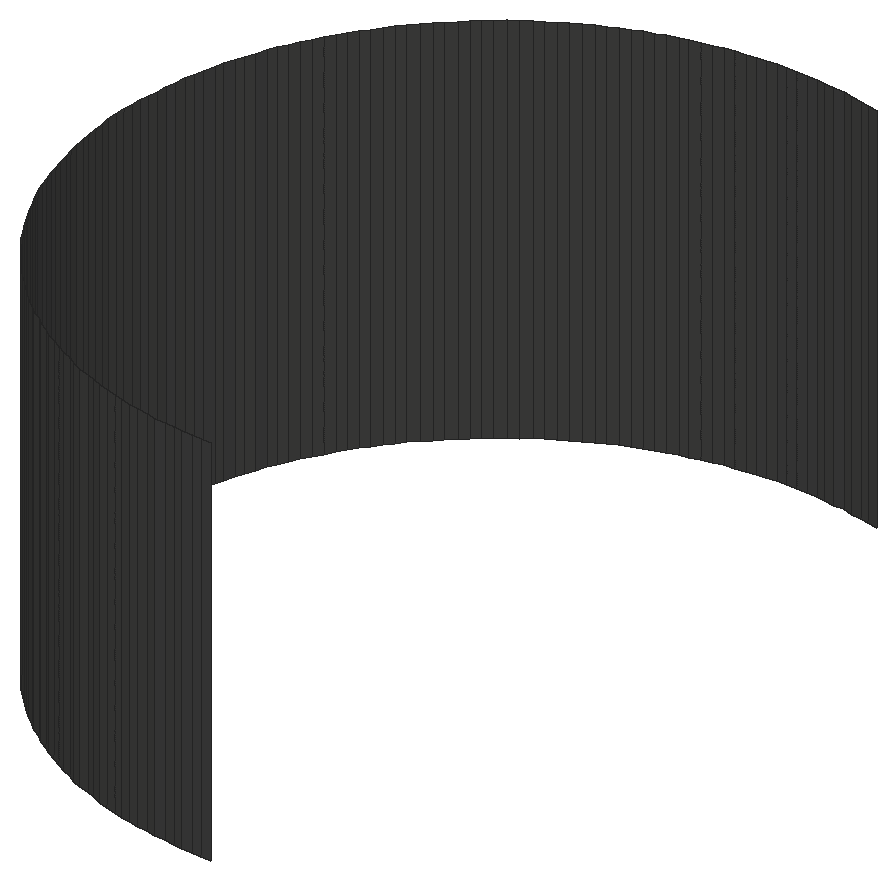
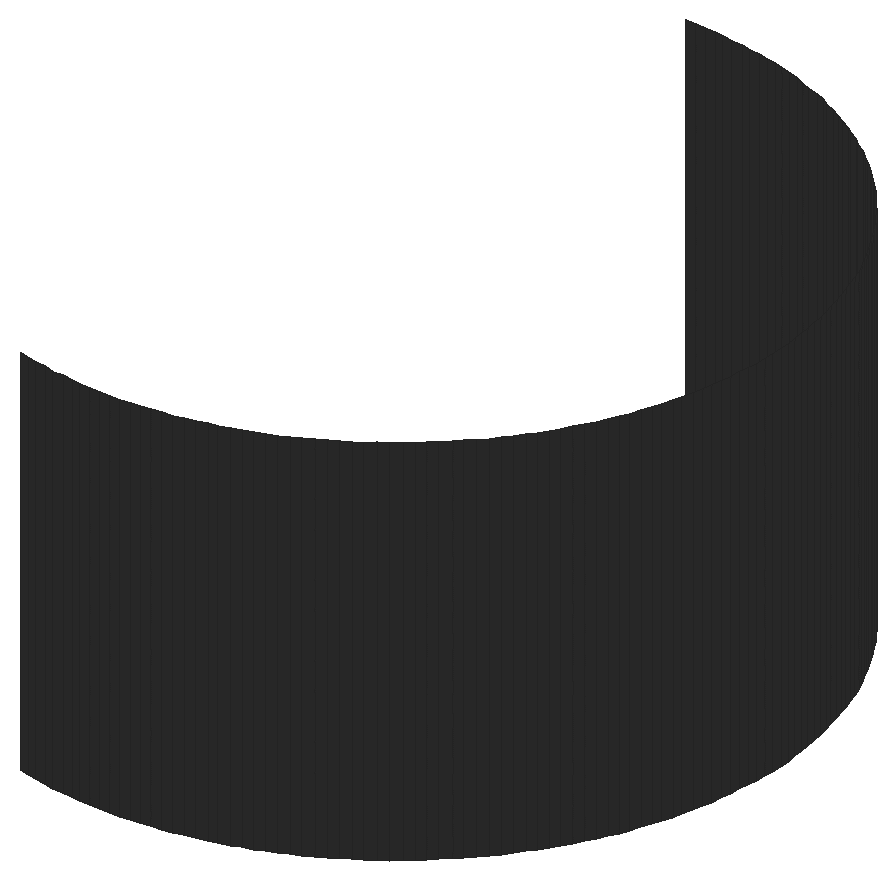
# SketchUp Ruby script. Lengths in inches.
U = 1.inch
M = Sketchup.active_model
def pt(a) = Geom::Point3d.new(a.map { |v| v * U })
def face(e, loops, mat)
  f = e.add_face(loops[0].map { |a| pt(a) })
  loops[1..].each { |l| e.add_face(l.map { |a| pt(a) }).erase! }
  f.material = f.back_material = mat if mat
  f
end
# faces: each face lists its corners as indices into pts; further lists are holes
def faces(e, pts, list, mat = nil) = list.each { |f| face(e, (f[0].is_a?(Array) ? f : [f]).map { |l| l.map { |i| pts[i] } }, mat) }
# xy, xz, yz: faces in a plane at the given z, y or x. An outline is a flat list of corners, or four numbers for a rectangle; further outlines are holes
def ring(l) = l.size == 4 ? [[l[0], l[1]], [l[2], l[1]], [l[2], l[3]], [l[0], l[3]]] : l.each_slice(2).to_a
def flat(e, list, mat, &to3) = list.each { |f| face(e, (f[0].is_a?(Array) ? f : [f]).map { |l| ring(l).map { |u, v| to3.(u, v) } }, mat) }
def xy(e, z, list, mat = nil) = flat(e, list, mat) { |x, y| [x, y, z] }
def xz(e, y, list, mat = nil) = flat(e, list, mat) { |x, z| [x, y, z] }
def yz(e, x, list, mat = nil) = flat(e, list, mat) { |y, z| [x, y, z] }
def lines(e, pts, list) = list.each { |a, b| e.add_line(pt(pts[a]), pt(pts[b])) }
# prism: a flat outline (further loops are holes) pulled along v
def prism(e, loops, v, mat = nil)
  f = face(e, loops, mat); d = Geom::Vector3d.new(v.map { |x| x * U })
  f.pushpull(f.normal.samedirection?(d) ? d.length : -d.length)
end
def box(e, o, s, mat = nil) = prism(e, [[o, [o[0] + s[0], o[1], o[2]], [o[0] + s[0], o[1] + s[1], o[2]], [o[0], o[1] + s[1], o[2]]]], [0, 0, s[2]], mat)
def at(x, y, z, deg = 0) = Geom::Transformation.translation(pt([x, y, z])) * Geom::Transformation.rotation(ORIGIN, Z_AXIS, deg.degrees)
def axes(o, x, y, z) = Geom::Transformation.new([*x, 0, *y, 0, *z, 0, *pt(o).to_a, 1])
def part(name) = M.definitions.add(name)
# library, detail: a bought-in or finely detailed component or shape, given as its bounding box
def library(name, o, s) = part(name).tap { |d| box(d.entities, o, s) }
def detail(e, o, s) = box(e.add_group.entities, o, s)
def put(e, d, t, mat = nil) = e.add_instance(d, t).tap { |i| i.material = mat if mat }
def group(e, t, mat = nil) = e.add_group.tap { |g| g.transformation = t; g.material = mat if mat }.entities
root = M.entities
M.materials.add("1448 AP 8253 RAVEN SONG").color = [64, 64, 63]
xz(root,217.5,[[117.99,471,118.07,474],[118.07,471,118.15,474],[118.15,471,118.23,474]],"1448 AP 8253 RAVEN SONG")
xz(root,217.52,[[117.76,471,117.84,474]],"1448 AP 8253 RAVEN SONG")
xz(root,223.48,[[118.44,471,118.52,474]],"1448 AP 8253 RAVEN SONG")
xz(root,223.5,[[117.97,471,118.05,474],[118.05,471,118.13,474],[118.13,471,118.21,474],[118.21,471,118.29,474]],"1448 AP 8253 RAVEN SONG")
yz(root,115.14,[[220.33,471,220.41,474],[220.41,471,220.49,474],[220.49,471,220.57,474],[220.57,471,220.65,474]],"1448 AP 8253 RAVEN SONG")
yz(root,115.16,[[220.8,471,220.88,474]],"1448 AP 8253 RAVEN SONG")
p = [[117.6,217.55,471],[117.53,217.5625,471],[117.53,217.5625,474],[117.6,217.55,474],[117.68,217.54,471],[117.68,217.54,474],
  [117.76,217.52,471],[117.76,217.52,474],[117.92,217.51,471],[117.84,217.52,471],[117.84,217.52,474],[117.92,217.51,474],
  [117.99,217.5,471],[117.99,217.5,474],[117.22,217.64,471],[117.15,217.67,471],[117.15,217.67,474],[117.22,217.64,474],
  [117.3,217.62,471],[117.3,217.62,474],[117.375,217.6,471],[117.375,217.6,474],[117.45,217.58,471],[117.45,217.58,474],
  [117,217.72,471],[116.93,217.75,471],[116.93,217.75,474],[117,217.72,474],[117.08,217.7,471],[117.08,217.7,474],
  [116.79,217.82,471],[116.72,217.86,471],[116.72,217.86,474],[116.79,217.82,474],[116.86,217.79,471],[116.86,217.79,474],
  [116.58,217.9375,471],[116.52,217.98,471],[116.52,217.98,474],[116.58,217.9375,474],[116.65,217.9,471],[116.65,217.9,474],
  [116.45,218.02,471],[116.39,218.07,471],[116.39,218.07,474],[116.45,218.02,474],[116.32,218.11,471],[116.32,218.11,474],
  [116.26,218.16,471],[116.26,218.16,474],[116.2,218.21,471],[116.14,218.26,471],[116.14,218.26,474],[116.2,218.21,474],
  [116.08,218.32,471],[116.03,218.37,471],[116.03,218.37,474],[116.08,218.32,474],[115.97,218.43,471],[115.92,218.48,471],
  [115.92,218.48,474],[115.97,218.43,474],[115.87,218.54,471],[115.82,218.6,471],[115.82,218.6,474],[115.87,218.54,474],
  [115.77,218.66,471],[115.77,218.66,474],[115.72,218.73,471],[115.72,218.73,474],[115.67,218.79,471],[115.67,218.79,474],
  [115.63,218.86,471],[115.63,218.86,474],[115.59,218.92,471],[115.55,218.99,471],[115.55,218.99,474],[115.59,218.92,474],
  [115.51,219.06,471],[115.51,219.06,474],[115.47,219.13,471],[115.4375,219.2,471],[115.4375,219.2,474],[115.47,219.13,474],
  [115.4,219.27,471],[115.4,219.27,474],[115.37,219.34,471],[115.34,219.41,471],[115.34,219.41,474],[115.37,219.34,474],
  [115.32,219.49,471],[115.32,219.49,474],[115.29,219.5625,471],[115.29,219.5625,474],[115.27,219.64,471],[115.25,219.71,471],
  [115.25,219.71,474],[115.27,219.64,474],[115.23,219.79,471],[115.23,219.79,474],[115.21,219.87,471],[115.21,219.87,474],
  [115.19,219.94,471],[115.19,219.94,474],[115.18,220.02,471],[115.18,220.02,474],[115.17,220.1,471],[115.17,220.1,474],
  [115.16,220.18,471],[115.16,220.18,474],[115.15,220.25,471],[115.15,220.25,474],[115.14,220.33,471],[115.14,220.33,474],
  [115.14,220.65,471],[115.15,220.72,471],[115.15,220.72,474],[115.14,220.65,474],[115.16,220.8,471],[115.16,220.8,474],
  [115.16,220.88,471],[115.18,220.96,471],[115.18,220.96,474],[115.16,220.88,474],[115.1875,221.04,471],[115.1875,221.04,474],
  [115.2,221.11,471],[115.2,221.11,474],[115.22,221.1875,471],[115.22,221.1875,474],[115.24,221.27,471],[115.24,221.27,474],
  [115.26,221.34,471],[115.26,221.34,474],[115.28,221.42,471],[115.28,221.42,474],[115.31,221.49,471],[115.31,221.49,474],
  [115.34,221.5625,471],[115.34,221.5625,474],[115.36,221.64,471],[115.36,221.64,474],[115.39,221.71,471],[115.39,221.71,474],
  [115.43,221.78,471],[115.43,221.78,474],[115.46,221.85,471],[115.46,221.85,474],[115.5,221.92,471],[115.5,221.92,474],
  [115.54,221.99,471],[115.54,221.99,474],[115.58,222.06,471],[115.58,222.06,474],[115.62,222.125,471],[115.62,222.125,474],
  [115.66,222.19,471],[115.66,222.19,474],[115.71,222.25,471],[115.71,222.25,474],[115.75,222.32,471],[115.75,222.32,474],
  [115.8,222.38,471],[115.8,222.38,474],[115.85,222.44,471],[115.85,222.44,474],[115.9,222.5,471],[115.9,222.5,474],
  [115.96,222.56,471],[115.96,222.56,474],[116.01,222.61,471],[116.01,222.61,474],[116.07,222.67,471],[116.07,222.67,474],
  [116.125,222.72,471],[116.125,222.72,474],[116.18,222.77,471],[116.18,222.77,474],[116.24,222.82,471],[116.24,222.82,474],
  [116.3,222.875,471],[116.3,222.875,474],[116.37,222.92,471],[116.37,222.92,474],[116.43,222.97,471],[116.43,222.97,474],
  [116.5,223.01,471],[116.5,223.01,474],[116.5625,223.05,471],[116.5625,223.05,474],[116.63,223.09,471],[116.63,223.09,474],
  [116.7,223.13,471],[116.7,223.13,474],[116.77,223.17,471],[116.77,223.17,474],[116.84,223.2,471],[116.84,223.2,474],
  [116.91,223.24,471],[116.91,223.24,474],[116.98,223.27,471],[116.98,223.27,474],[117.05,223.3,471],[117.05,223.3,474],
  [117.13,223.32,471],[117.13,223.32,474],[117.2,223.35,471],[117.2,223.35,474],[117.28,223.375,471],[117.28,223.375,474],
  [117.35,223.39,471],[117.35,223.39,474],[117.43,223.41,471],[117.43,223.41,474],[117.51,223.43,471],[117.51,223.43,474],
  [117.58,223.45,471],[117.58,223.45,474],[117.66,223.46,471],[117.66,223.46,474],[118.68,223.45,471],[118.75,223.4375,471],
  [118.75,223.4375,474],[118.68,223.45,474],[118.83,223.42,471],[118.83,223.42,474],[117.74,223.47,471],[117.74,223.47,474],
  [117.82,223.48,471],[117.82,223.48,474],[117.89,223.49,471],[117.89,223.49,474],[117.97,223.5,471],[117.97,223.5,474],
  [118.29,223.5,471],[118.36,223.49,471],[118.36,223.49,474],[118.29,223.5,474],[118.44,223.48,471],[118.44,223.48,474],
  [118.52,223.48,471],[118.6,223.46,471],[118.6,223.46,474],[118.52,223.48,474]]
faces(root,p,[[0,1,2,3],[4,0,3,5],[6,4,5,7],[8,9,10,11],[12,8,11,13],[14,15,16,17],[18,14,17,19],[20,18,19,21],
  [22,20,21,23],[1,22,23,2],[24,25,26,27],[28,24,27,29],[15,28,29,16],[30,31,32,33],[34,30,33,35],[25,34,35,26],
  [36,37,38,39],[31,40,41,32],[40,36,39,41],[42,43,44,45],[37,42,45,38],[43,46,47,44],[46,48,49,47],[50,51,52,53],
  [48,50,53,49],[54,55,56,57],[51,54,57,52],[58,59,60,61],[55,58,61,56],[62,63,64,65],[59,62,65,60],[63,66,67,64],
  [66,68,69,67],[68,70,71,69],[70,72,73,71],[74,75,76,77],[72,74,77,73],[75,78,79,76],[80,81,82,83],[78,80,83,79],
  [81,84,85,82],[86,87,88,89],[84,86,89,85],[87,90,91,88],[90,92,93,91],[94,95,96,97],[92,94,97,93],[95,98,99,96],
  [98,100,101,99],[100,102,103,101],[102,104,105,103],[104,106,107,105],[106,108,109,107],[108,110,111,109],[110,112,113,111],[114,115,116,117],
  [115,118,119,116],[120,121,122,123],[121,124,125,122],[124,126,127,125],[126,128,129,127],[128,130,131,129],[130,132,133,131],[132,134,135,133],
  [134,136,137,135],[136,138,139,137],[138,140,141,139],[140,142,143,141],[142,144,145,143],[144,146,147,145],[146,148,149,147],[148,150,151,149],
  [150,152,153,151],[152,154,155,153],[154,156,157,155],[156,158,159,157],[158,160,161,159],[160,162,163,161],[162,164,165,163],[164,166,167,165],
  [166,168,169,167],[168,170,171,169],[170,172,173,171],[172,174,175,173],[174,176,177,175],[176,178,179,177],[178,180,181,179],[180,182,183,181],
  [182,184,185,183],[184,186,187,185],[186,188,189,187],[188,190,191,189],[190,192,193,191],[192,194,195,193],[194,196,197,195],[196,198,199,197],
  [198,200,201,199],[200,202,203,201],[202,204,205,203],[204,206,207,205],[206,208,209,207],[208,210,211,209],[210,212,213,211],[212,214,215,213],
  [214,216,217,215],[216,218,219,217],[220,221,222,223],[221,224,225,222],[218,226,227,219],[226,228,229,227],[228,230,231,229],[230,232,233,231],
  [234,235,236,237],[235,238,239,236],[240,241,242,243],[241,220,223,242]],"1448 AP 8253 RAVEN SONG")
